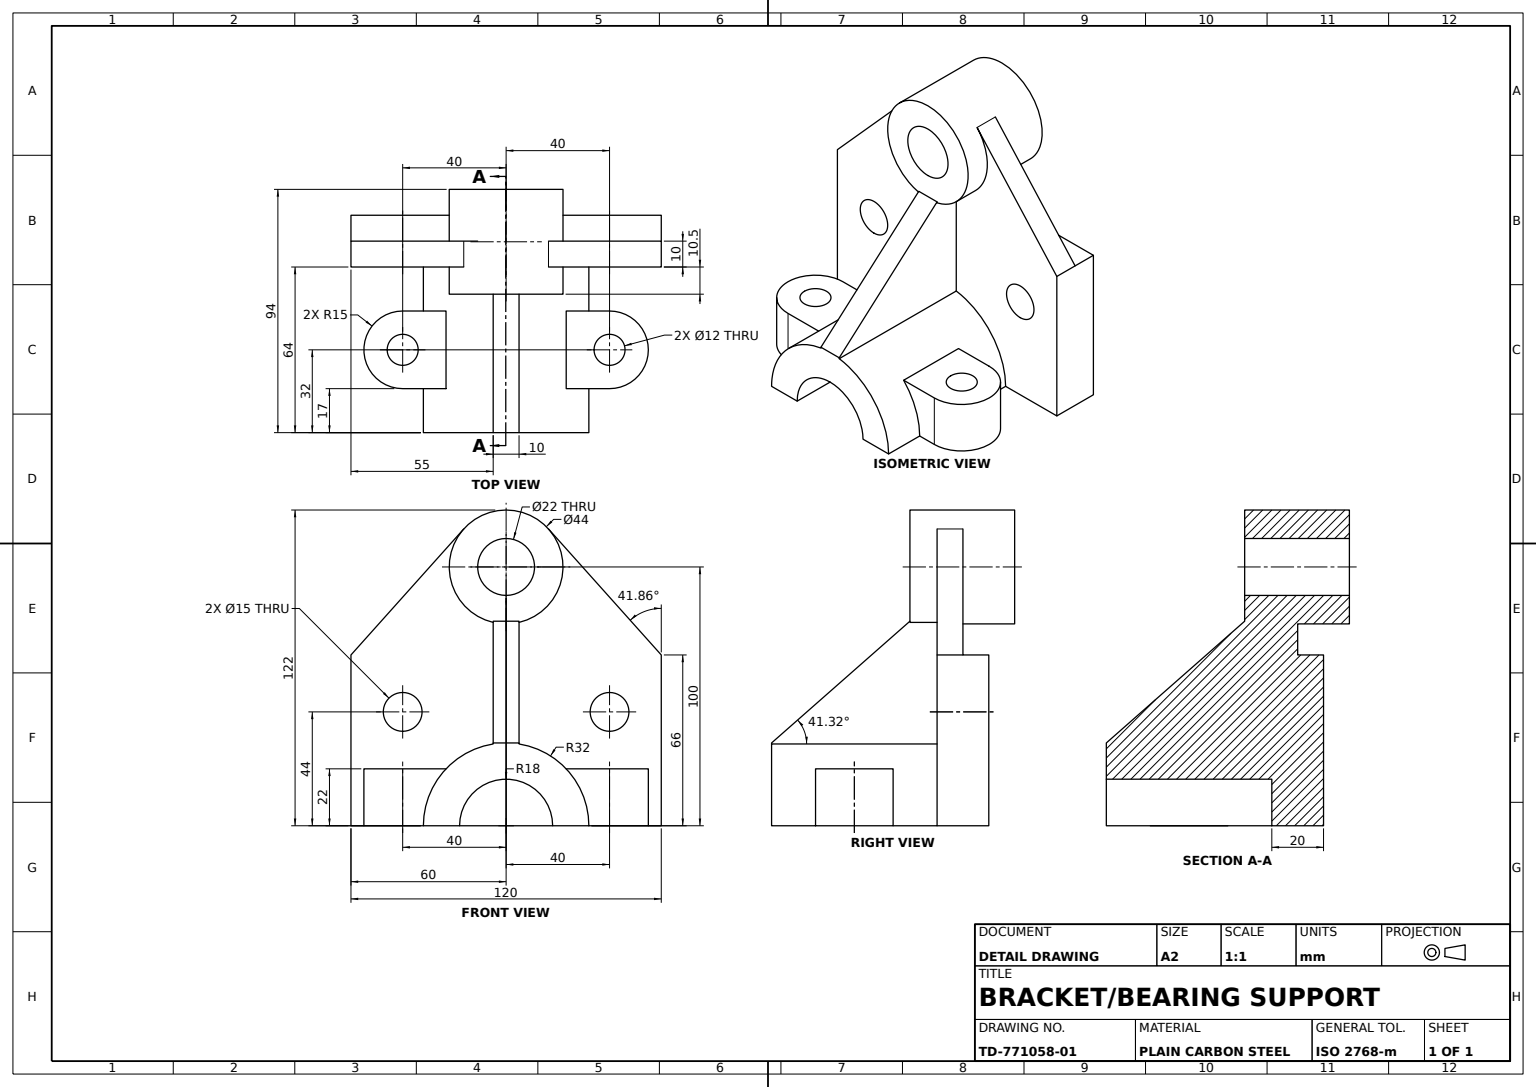
ISO-10303-21;
HEADER;
FILE_DESCRIPTION((''),'2;1');
FILE_NAME('','',(''),(''),'','','');
FILE_SCHEMA(('AUTOMOTIVE_DESIGN'));
ENDSEC;
DATA;
#1=APPLICATION_CONTEXT('');
#2=PRODUCT_CONTEXT('',#1,'mechanical');
#3=PRODUCT('','','',(#2));
#4=PRODUCT_DEFINITION_FORMATION('','',#3);
#5=PRODUCT_DEFINITION_CONTEXT('',#1,'design');
#6=PRODUCT_DEFINITION('','',#4,#5);
#7=PRODUCT_DEFINITION_SHAPE('','',#6);
#8=(LENGTH_UNIT()NAMED_UNIT(*)SI_UNIT(.MILLI.,.METRE.));
#9=(NAMED_UNIT(*)PLANE_ANGLE_UNIT()SI_UNIT($,.RADIAN.));
#10=(NAMED_UNIT(*)SI_UNIT($,.STERADIAN.)SOLID_ANGLE_UNIT());
#11=UNCERTAINTY_MEASURE_WITH_UNIT(LENGTH_MEASURE(1.E-05),#8,'distance_accuracy_value','');
#12=(GEOMETRIC_REPRESENTATION_CONTEXT(3)GLOBAL_UNCERTAINTY_ASSIGNED_CONTEXT((#11))GLOBAL_UNIT_ASSIGNED_CONTEXT((#8,#9,#10))REPRESENTATION_CONTEXT('',''));
#13=CARTESIAN_POINT('',(-10.,3.5,100.));
#14=VERTEX_POINT('',#13);
#15=CARTESIAN_POINT('',(-10.,18.5,100.));
#16=VERTEX_POINT('',#15);
#17=CARTESIAN_POINT('',(-10.,11.,100.));
#18=DIRECTION('',(1.,0.,0.));
#19=DIRECTION('',(0.,1.,0.));
#20=AXIS2_PLACEMENT_3D('',#17,#18,#19);
#21=CIRCLE('',#20,7.5);
#22=EDGE_CURVE('',#14,#16,#21,.T.);
#23=ORIENTED_EDGE('',*,*,#22,.F.);
#24=CARTESIAN_POINT('',(10.,3.5,100.));
#25=VERTEX_POINT('',#24);
#26=CARTESIAN_POINT('',(-20.,3.5,100.));
#27=VECTOR('',#18,1000.);
#28=LINE('',#26,#27);
#29=EDGE_CURVE('',#14,#25,#28,.T.);
#30=ORIENTED_EDGE('',*,*,#29,.T.);
#31=CARTESIAN_POINT('',(10.,18.5,100.));
#32=VERTEX_POINT('',#31);
#33=CARTESIAN_POINT('',(10.,11.,100.));
#34=AXIS2_PLACEMENT_3D('',#33,#18,#19);
#35=CIRCLE('',#34,7.5);
#36=EDGE_CURVE('',#25,#32,#35,.T.);
#37=ORIENTED_EDGE('',*,*,#36,.T.);
#38=CARTESIAN_POINT('',(-20.,18.5,100.));
#39=LINE('',#38,#27);
#40=EDGE_CURVE('',#16,#32,#39,.T.);
#41=ORIENTED_EDGE('',*,*,#40,.F.);
#42=EDGE_LOOP('',(#23,#30,#37,#41));
#43=FACE_OUTER_BOUND('',#42,.T.);
#44=CARTESIAN_POINT('',(-20.,11.,100.));
#45=AXIS2_PLACEMENT_3D('',#44,#18,#19);
#46=CYLINDRICAL_SURFACE('',#45,7.5);
#47=ADVANCED_FACE('',(#43),#46,.F.);
#48=CARTESIAN_POINT('',(74.,-1.393039,65.));
#49=VERTEX_POINT('',#48);
#50=CARTESIAN_POINT('',(74.,-33.,92.));
#51=VERTEX_POINT('',#50);
#52=CARTESIAN_POINT('',(74.,-33.,60.));
#53=AXIS2_PLACEMENT_3D('',#52,#18,#19);
#54=CIRCLE('',#53,32.);
#55=EDGE_CURVE('',#49,#51,#54,.T.);
#56=ORIENTED_EDGE('',*,*,#55,.F.);
#57=CARTESIAN_POINT('',(10.,-1.393039,65.));
#58=VERTEX_POINT('',#57);
#59=DIRECTION('',(-1.,0.,0.));
#60=VECTOR('',#59,1000.);
#61=LINE('',#48,#60);
#62=EDGE_CURVE('',#49,#58,#61,.T.);
#63=ORIENTED_EDGE('',*,*,#62,.T.);
#64=CARTESIAN_POINT('',(10.,-33.,92.));
#65=VERTEX_POINT('',#64);
#66=CARTESIAN_POINT('',(10.,-33.,60.));
#67=AXIS2_PLACEMENT_3D('',#66,#18,#19);
#68=CIRCLE('',#67,32.);
#69=EDGE_CURVE('',#58,#65,#68,.T.);
#70=ORIENTED_EDGE('',*,*,#69,.T.);
#71=CARTESIAN_POINT('',(27.,-33.,92.));
#72=VERTEX_POINT('',#71);
#73=LINE('',#50,#60);
#74=EDGE_CURVE('',#72,#65,#73,.T.);
#75=ORIENTED_EDGE('',*,*,#74,.F.);
#76=CARTESIAN_POINT('',(27.,-11.,83.2379));
#77=VERTEX_POINT('',#76);
#78=CARTESIAN_POINT('',(27.,-33.,60.));
#79=DIRECTION('',(0.,0.,1.));
#80=AXIS2_PLACEMENT_3D('',#78,#59,#79);
#81=CIRCLE('',#80,32.);
#82=EDGE_CURVE('',#72,#77,#81,.T.);
#83=ORIENTED_EDGE('',*,*,#82,.T.);
#84=CARTESIAN_POINT('',(57.,-11.,83.2379));
#85=VERTEX_POINT('',#84);
#86=CARTESIAN_POINT('',(74.,-11.,83.2379));
#87=LINE('',#86,#60);
#88=EDGE_CURVE('',#85,#77,#87,.T.);
#89=ORIENTED_EDGE('',*,*,#88,.F.);
#90=CARTESIAN_POINT('',(57.,-33.,92.));
#91=VERTEX_POINT('',#90);
#92=CARTESIAN_POINT('',(57.,-33.,60.));
#93=DIRECTION('',(0.,0.,-1.));
#94=AXIS2_PLACEMENT_3D('',#92,#18,#93);
#95=CIRCLE('',#94,32.);
#96=EDGE_CURVE('',#85,#91,#95,.T.);
#97=ORIENTED_EDGE('',*,*,#96,.T.);
#98=EDGE_CURVE('',#51,#91,#73,.T.);
#99=ORIENTED_EDGE('',*,*,#98,.F.);
#100=EDGE_LOOP('',(#56,#63,#70,#75,#83,#89,#97,#99));
#101=FACE_OUTER_BOUND('',#100,.T.);
#102=DIRECTION('',(0.,-1.,0.));
#103=AXIS2_PLACEMENT_3D('',#52,#59,#102);
#104=CYLINDRICAL_SURFACE('',#103,32.);
#105=ADVANCED_FACE('',(#101),#104,.T.);
#106=CARTESIAN_POINT('',(57.,-33.,28.));
#107=VERTEX_POINT('',#106);
#108=CARTESIAN_POINT('',(57.,-11.,36.7621));
#109=VERTEX_POINT('',#108);
#110=EDGE_CURVE('',#107,#109,#95,.T.);
#111=ORIENTED_EDGE('',*,*,#110,.F.);
#112=CARTESIAN_POINT('',(57.,-33.,20.));
#113=VERTEX_POINT('',#112);
#114=CARTESIAN_POINT('',(57.,-33.,38.));
#115=VECTOR('',#79,1000.);
#116=LINE('',#114,#115);
#117=EDGE_CURVE('',#113,#107,#116,.T.);
#118=ORIENTED_EDGE('',*,*,#117,.F.);
#119=CARTESIAN_POINT('',(57.,-11.,20.));
#120=VERTEX_POINT('',#119);
#121=VECTOR('',#102,1000.);
#122=LINE('',#119,#121);
#123=EDGE_CURVE('',#120,#113,#122,.T.);
#124=ORIENTED_EDGE('',*,*,#123,.F.);
#125=CARTESIAN_POINT('',(57.,-11.,35.));
#126=LINE('',#125,#115);
#127=EDGE_CURVE('',#120,#109,#126,.T.);
#128=ORIENTED_EDGE('',*,*,#127,.T.);
#129=EDGE_LOOP('',(#111,#118,#124,#128));
#130=FACE_OUTER_BOUND('',#129,.T.);
#131=CARTESIAN_POINT('',(57.,-11.,38.));
#132=AXIS2_PLACEMENT_3D('',#131,#18,#93);
#133=PLANE('',#132);
#134=ADVANCED_FACE('',(#130),#133,.T.);
#135=CARTESIAN_POINT('',(42.,-33.,5.));
#136=VERTEX_POINT('',#135);
#137=CARTESIAN_POINT('',(42.,-33.,20.));
#138=AXIS2_PLACEMENT_3D('',#137,#102,#93);
#139=CIRCLE('',#138,15.);
#140=EDGE_CURVE('',#136,#113,#139,.T.);
#141=ORIENTED_EDGE('',*,*,#140,.T.);
#142=ORIENTED_EDGE('',*,*,#117,.T.);
#143=CARTESIAN_POINT('',(74.,-33.,28.));
#144=VERTEX_POINT('',#143);
#145=LINE('',#143,#60);
#146=EDGE_CURVE('',#144,#107,#145,.T.);
#147=ORIENTED_EDGE('',*,*,#146,.F.);
#148=CARTESIAN_POINT('',(74.,-33.,42.));
#149=VERTEX_POINT('',#148);
#150=VECTOR('',#93,1000.);
#151=LINE('',#148,#150);
#152=EDGE_CURVE('',#149,#144,#151,.T.);
#153=ORIENTED_EDGE('',*,*,#152,.F.);
#154=CARTESIAN_POINT('',(10.,-33.,42.));
#155=VERTEX_POINT('',#154);
#156=LINE('',#148,#60);
#157=EDGE_CURVE('',#149,#155,#156,.T.);
#158=ORIENTED_EDGE('',*,*,#157,.T.);
#159=CARTESIAN_POINT('',(10.,-33.,78.));
#160=VERTEX_POINT('',#159);
#161=CARTESIAN_POINT('',(10.,-33.,120.));
#162=LINE('',#161,#150);
#163=EDGE_CURVE('',#160,#155,#162,.T.);
#164=ORIENTED_EDGE('',*,*,#163,.F.);
#165=CARTESIAN_POINT('',(74.,-33.,78.));
#166=VERTEX_POINT('',#165);
#167=LINE('',#165,#60);
#168=EDGE_CURVE('',#166,#160,#167,.T.);
#169=ORIENTED_EDGE('',*,*,#168,.F.);
#170=LINE('',#50,#150);
#171=EDGE_CURVE('',#51,#166,#170,.T.);
#172=ORIENTED_EDGE('',*,*,#171,.F.);
#173=ORIENTED_EDGE('',*,*,#98,.T.);
#174=CARTESIAN_POINT('',(57.,-33.,100.));
#175=VERTEX_POINT('',#174);
#176=CARTESIAN_POINT('',(57.,-33.,85.));
#177=LINE('',#176,#115);
#178=EDGE_CURVE('',#91,#175,#177,.T.);
#179=ORIENTED_EDGE('',*,*,#178,.T.);
#180=CARTESIAN_POINT('',(27.,-33.,100.));
#181=VERTEX_POINT('',#180);
#182=CARTESIAN_POINT('',(42.,-33.,100.));
#183=AXIS2_PLACEMENT_3D('',#182,#102,#93);
#184=CIRCLE('',#183,15.);
#185=EDGE_CURVE('',#175,#181,#184,.T.);
#186=ORIENTED_EDGE('',*,*,#185,.T.);
#187=LINE('',#180,#150);
#188=EDGE_CURVE('',#181,#72,#187,.T.);
#189=ORIENTED_EDGE('',*,*,#188,.T.);
#190=ORIENTED_EDGE('',*,*,#74,.T.);
#191=VERTEX_POINT('',#161);
#192=EDGE_CURVE('',#191,#65,#162,.T.);
#193=ORIENTED_EDGE('',*,*,#192,.F.);
#194=CARTESIAN_POINT('',(-10.,-33.,120.));
#195=VERTEX_POINT('',#194);
#196=LINE('',#194,#27);
#197=EDGE_CURVE('',#195,#191,#196,.T.);
#198=ORIENTED_EDGE('',*,*,#197,.F.);
#199=CARTESIAN_POINT('',(-10.,-33.,0.));
#200=VERTEX_POINT('',#199);
#201=LINE('',#194,#150);
#202=EDGE_CURVE('',#195,#200,#201,.T.);
#203=ORIENTED_EDGE('',*,*,#202,.T.);
#204=CARTESIAN_POINT('',(10.,-33.,0.));
#205=VERTEX_POINT('',#204);
#206=LINE('',#199,#27);
#207=EDGE_CURVE('',#200,#205,#206,.T.);
#208=ORIENTED_EDGE('',*,*,#207,.T.);
#209=CARTESIAN_POINT('',(10.,-33.,28.));
#210=VERTEX_POINT('',#209);
#211=EDGE_CURVE('',#210,#205,#162,.T.);
#212=ORIENTED_EDGE('',*,*,#211,.F.);
#213=CARTESIAN_POINT('',(27.,-33.,28.));
#214=VERTEX_POINT('',#213);
#215=EDGE_CURVE('',#214,#210,#145,.T.);
#216=ORIENTED_EDGE('',*,*,#215,.F.);
#217=CARTESIAN_POINT('',(27.,-33.,20.));
#218=VERTEX_POINT('',#217);
#219=LINE('',#217,#150);
#220=EDGE_CURVE('',#214,#218,#219,.T.);
#221=ORIENTED_EDGE('',*,*,#220,.T.);
#222=EDGE_CURVE('',#218,#136,#139,.T.);
#223=ORIENTED_EDGE('',*,*,#222,.T.);
#224=EDGE_LOOP('',(#141,#142,#147,#153,#158,#164,#169,#172,#173,#179,#186,#189,#190,#193,#198,#203,#208,#212,#216,#221,#223));
#225=FACE_OUTER_BOUND('',#224,.T.);
#226=CARTESIAN_POINT('',(42.,-33.,26.));
#227=VERTEX_POINT('',#226);
#228=CARTESIAN_POINT('',(42.,-33.,14.));
#229=VERTEX_POINT('',#228);
#230=CIRCLE('',#138,6.);
#231=EDGE_CURVE('',#227,#229,#230,.T.);
#232=ORIENTED_EDGE('',*,*,#231,.F.);
#233=EDGE_CURVE('',#229,#227,#230,.T.);
#234=ORIENTED_EDGE('',*,*,#233,.F.);
#235=EDGE_LOOP('',(#232,#234));
#236=FACE_BOUND('',#235,.T.);
#237=CARTESIAN_POINT('',(42.,-33.,94.));
#238=VERTEX_POINT('',#237);
#239=CARTESIAN_POINT('',(42.,-33.,106.));
#240=VERTEX_POINT('',#239);
#241=CIRCLE('',#183,6.);
#242=EDGE_CURVE('',#238,#240,#241,.T.);
#243=ORIENTED_EDGE('',*,*,#242,.F.);
#244=EDGE_CURVE('',#240,#238,#241,.T.);
#245=ORIENTED_EDGE('',*,*,#244,.F.);
#246=EDGE_LOOP('',(#243,#245));
#247=FACE_BOUND('',#246,.T.);
#248=AXIS2_PLACEMENT_3D('',#194,#19,#79);
#249=PLANE('',#248);
#250=ADVANCED_FACE('',(#225,#236,#247),#249,.F.);
#251=CARTESIAN_POINT('',(10.,33.,120.));
#252=VERTEX_POINT('',#251);
#253=CARTESIAN_POINT('',(10.,81.680385,76.385551));
#254=VERTEX_POINT('',#253);
#255=CARTESIAN_POINT('',(10.,74.333671,82.967728));
#256=DIRECTION('',(0.,0.744797795,-0.667290226));
#257=VECTOR('',#256,1000.);
#258=LINE('',#255,#257);
#259=EDGE_CURVE('',#252,#254,#258,.T.);
#260=ORIENTED_EDGE('',*,*,#259,.T.);
#261=CARTESIAN_POINT('',(0.,81.680385,76.385551));
#262=VERTEX_POINT('',#261);
#263=LINE('',#261,#27);
#264=EDGE_CURVE('',#262,#254,#263,.T.);
#265=ORIENTED_EDGE('',*,*,#264,.F.);
#266=CARTESIAN_POINT('',(0.,33.,120.));
#267=VERTEX_POINT('',#266);
#268=CARTESIAN_POINT('',(0.,74.333671,82.967728));
#269=LINE('',#268,#257);
#270=EDGE_CURVE('',#267,#262,#269,.T.);
#271=ORIENTED_EDGE('',*,*,#270,.F.);
#272=CARTESIAN_POINT('',(-10.,33.,120.));
#273=LINE('',#272,#60);
#274=EDGE_CURVE('',#252,#267,#273,.T.);
#275=ORIENTED_EDGE('',*,*,#274,.F.);
#276=EDGE_LOOP('',(#260,#265,#271,#275));
#277=FACE_OUTER_BOUND('',#276,.T.);
#278=DIRECTION('',(0.,-0.667290226,-0.744797795));
#279=AXIS2_PLACEMENT_3D('',#268,#278,#256);
#280=PLANE('',#279);
#281=ADVANCED_FACE('',(#277),#280,.F.);
#282=CARTESIAN_POINT('',(-10.,3.5,20.));
#283=VERTEX_POINT('',#282);
#284=CARTESIAN_POINT('',(-10.,18.5,20.));
#285=VERTEX_POINT('',#284);
#286=CARTESIAN_POINT('',(-10.,11.,20.));
#287=AXIS2_PLACEMENT_3D('',#286,#18,#19);
#288=CIRCLE('',#287,7.5);
#289=EDGE_CURVE('',#283,#285,#288,.T.);
#290=ORIENTED_EDGE('',*,*,#289,.F.);
#291=CARTESIAN_POINT('',(10.,3.5,20.));
#292=VERTEX_POINT('',#291);
#293=CARTESIAN_POINT('',(-20.,3.5,20.));
#294=LINE('',#293,#27);
#295=EDGE_CURVE('',#283,#292,#294,.T.);
#296=ORIENTED_EDGE('',*,*,#295,.T.);
#297=CARTESIAN_POINT('',(10.,18.5,20.));
#298=VERTEX_POINT('',#297);
#299=CARTESIAN_POINT('',(10.,11.,20.));
#300=AXIS2_PLACEMENT_3D('',#299,#18,#19);
#301=CIRCLE('',#300,7.5);
#302=EDGE_CURVE('',#292,#298,#301,.T.);
#303=ORIENTED_EDGE('',*,*,#302,.T.);
#304=CARTESIAN_POINT('',(-20.,18.5,20.));
#305=LINE('',#304,#27);
#306=EDGE_CURVE('',#285,#298,#305,.T.);
#307=ORIENTED_EDGE('',*,*,#306,.F.);
#308=EDGE_LOOP('',(#290,#296,#303,#307));
#309=FACE_OUTER_BOUND('',#308,.T.);
#310=CARTESIAN_POINT('',(-20.,11.,20.));
#311=AXIS2_PLACEMENT_3D('',#310,#18,#19);
#312=CYLINDRICAL_SURFACE('',#311,7.5);
#313=ADVANCED_FACE('',(#309),#312,.F.);
#314=CARTESIAN_POINT('',(42.,-11.,94.));
#315=VERTEX_POINT('',#314);
#316=CARTESIAN_POINT('',(42.,-11.,106.));
#317=VERTEX_POINT('',#316);
#318=CARTESIAN_POINT('',(42.,-11.,100.));
#319=AXIS2_PLACEMENT_3D('',#318,#102,#93);
#320=CIRCLE('',#319,6.);
#321=EDGE_CURVE('',#315,#317,#320,.T.);
#322=ORIENTED_EDGE('',*,*,#321,.T.);
#323=EDGE_CURVE('',#317,#315,#320,.T.);
#324=ORIENTED_EDGE('',*,*,#323,.T.);
#325=EDGE_LOOP('',(#322,#324));
#326=FACE_BOUND('',#325,.T.);
#327=CARTESIAN_POINT('',(27.,-11.,100.));
#328=VERTEX_POINT('',#327);
#329=LINE('',#327,#150);
#330=EDGE_CURVE('',#328,#77,#329,.T.);
#331=ORIENTED_EDGE('',*,*,#330,.F.);
#332=CARTESIAN_POINT('',(57.,-11.,100.));
#333=VERTEX_POINT('',#332);
#334=CIRCLE('',#319,15.);
#335=EDGE_CURVE('',#333,#328,#334,.T.);
#336=ORIENTED_EDGE('',*,*,#335,.F.);
#337=CARTESIAN_POINT('',(57.,-11.,83.));
#338=LINE('',#337,#115);
#339=EDGE_CURVE('',#85,#333,#338,.T.);
#340=ORIENTED_EDGE('',*,*,#339,.F.);
#341=ORIENTED_EDGE('',*,*,#88,.T.);
#342=EDGE_LOOP('',(#331,#336,#340,#341));
#343=FACE_OUTER_BOUND('',#342,.T.);
#344=PLANE('',#319);
#345=ADVANCED_FACE('',(#326,#343),#344,.F.);
#346=CARTESIAN_POINT('',(-20.,45.,60.));
#347=VERTEX_POINT('',#346);
#348=CARTESIAN_POINT('',(0.,45.,60.));
#349=VERTEX_POINT('',#348);
#350=LINE('',#348,#27);
#351=EDGE_CURVE('',#347,#349,#350,.T.);
#352=ORIENTED_EDGE('',*,*,#351,.T.);
#353=CARTESIAN_POINT('',(0.,67.,60.));
#354=AXIS2_PLACEMENT_3D('',#353,#59,#19);
#355=CIRCLE('',#354,22.);
#356=EDGE_CURVE('',#349,#262,#355,.T.);
#357=ORIENTED_EDGE('',*,*,#356,.T.);
#358=ORIENTED_EDGE('',*,*,#264,.T.);
#359=CARTESIAN_POINT('',(10.,45.575715,65.));
#360=VERTEX_POINT('',#359);
#361=CARTESIAN_POINT('',(10.,67.,60.));
#362=AXIS2_PLACEMENT_3D('',#361,#18,#19);
#363=CIRCLE('',#362,22.);
#364=EDGE_CURVE('',#254,#360,#363,.T.);
#365=ORIENTED_EDGE('',*,*,#364,.T.);
#366=CARTESIAN_POINT('',(20.5,45.575715,65.));
#367=VERTEX_POINT('',#366);
#368=CARTESIAN_POINT('',(0.,45.575715,65.));
#369=LINE('',#368,#60);
#370=EDGE_CURVE('',#367,#360,#369,.T.);
#371=ORIENTED_EDGE('',*,*,#370,.F.);
#372=CARTESIAN_POINT('',(20.5,89.,60.));
#373=VERTEX_POINT('',#372);
#374=CARTESIAN_POINT('',(20.5,67.,60.));
#375=AXIS2_PLACEMENT_3D('',#374,#18,#19);
#376=CIRCLE('',#375,22.);
#377=EDGE_CURVE('',#373,#367,#376,.T.);
#378=ORIENTED_EDGE('',*,*,#377,.F.);
#379=CARTESIAN_POINT('',(-20.,89.,60.));
#380=VERTEX_POINT('',#379);
#381=CARTESIAN_POINT('',(0.,89.,60.));
#382=LINE('',#381,#27);
#383=EDGE_CURVE('',#380,#373,#382,.T.);
#384=ORIENTED_EDGE('',*,*,#383,.F.);
#385=CARTESIAN_POINT('',(-20.,67.,60.));
#386=AXIS2_PLACEMENT_3D('',#385,#59,#102);
#387=CIRCLE('',#386,22.);
#388=EDGE_CURVE('',#347,#380,#387,.T.);
#389=ORIENTED_EDGE('',*,*,#388,.F.);
#390=EDGE_LOOP('',(#352,#357,#358,#365,#371,#378,#384,#389));
#391=FACE_OUTER_BOUND('',#390,.T.);
#392=AXIS2_PLACEMENT_3D('',#353,#18,#19);
#393=CYLINDRICAL_SURFACE('',#392,22.);
#394=ADVANCED_FACE('',(#391),#393,.T.);
#395=ORIENTED_EDGE('',*,*,#123,.T.);
#396=ORIENTED_EDGE('',*,*,#140,.F.);
#397=CARTESIAN_POINT('',(42.,-11.,5.));
#398=VERTEX_POINT('',#397);
#399=LINE('',#397,#121);
#400=EDGE_CURVE('',#398,#136,#399,.T.);
#401=ORIENTED_EDGE('',*,*,#400,.F.);
#402=CARTESIAN_POINT('',(42.,-11.,20.));
#403=AXIS2_PLACEMENT_3D('',#402,#102,#93);
#404=CIRCLE('',#403,15.);
#405=EDGE_CURVE('',#398,#120,#404,.T.);
#406=ORIENTED_EDGE('',*,*,#405,.T.);
#407=EDGE_LOOP('',(#395,#396,#401,#406));
#408=FACE_OUTER_BOUND('',#407,.T.);
#409=CYLINDRICAL_SURFACE('',#403,15.);
#410=ADVANCED_FACE('',(#408),#409,.T.);
#411=ORIENTED_EDGE('',*,*,#157,.F.);
#412=AXIS2_PLACEMENT_3D('',#52,#59,#19);
#413=CIRCLE('',#412,18.);
#414=EDGE_CURVE('',#166,#149,#413,.T.);
#415=ORIENTED_EDGE('',*,*,#414,.F.);
#416=ORIENTED_EDGE('',*,*,#168,.T.);
#417=AXIS2_PLACEMENT_3D('',#66,#59,#19);
#418=CIRCLE('',#417,18.);
#419=EDGE_CURVE('',#160,#155,#418,.T.);
#420=ORIENTED_EDGE('',*,*,#419,.T.);
#421=EDGE_LOOP('',(#411,#415,#416,#420));
#422=FACE_OUTER_BOUND('',#421,.T.);
#423=CYLINDRICAL_SURFACE('',#103,18.);
#424=ADVANCED_FACE('',(#422),#423,.F.);
#425=CARTESIAN_POINT('',(10.,45.575715,55.));
#426=VERTEX_POINT('',#425);
#427=CARTESIAN_POINT('',(10.,81.680385,43.614449));
#428=VERTEX_POINT('',#427);
#429=EDGE_CURVE('',#426,#428,#363,.T.);
#430=ORIENTED_EDGE('',*,*,#429,.F.);
#431=CARTESIAN_POINT('',(10.,-1.393039,55.));
#432=VERTEX_POINT('',#431);
#433=CARTESIAN_POINT('',(10.,-5.,55.));
#434=LINE('',#433,#121);
#435=EDGE_CURVE('',#426,#432,#434,.T.);
#436=ORIENTED_EDGE('',*,*,#435,.T.);
#437=EDGE_CURVE('',#210,#432,#68,.T.);
#438=ORIENTED_EDGE('',*,*,#437,.F.);
#439=ORIENTED_EDGE('',*,*,#211,.T.);
#440=CARTESIAN_POINT('',(10.,33.,0.));
#441=VERTEX_POINT('',#440);
#442=VECTOR('',#19,1000.);
#443=LINE('',#440,#442);
#444=EDGE_CURVE('',#205,#441,#443,.T.);
#445=ORIENTED_EDGE('',*,*,#444,.T.);
#446=CARTESIAN_POINT('',(10.,14.694116,-16.400878));
#447=DIRECTION('',(0.,0.744797795,0.667290226));
#448=VECTOR('',#447,1000.);
#449=LINE('',#446,#448);
#450=EDGE_CURVE('',#441,#428,#449,.T.);
#451=ORIENTED_EDGE('',*,*,#450,.T.);
#452=EDGE_LOOP('',(#430,#436,#438,#439,#445,#451));
#453=FACE_OUTER_BOUND('',#452,.T.);
#454=EDGE_CURVE('',#298,#292,#301,.T.);
#455=ORIENTED_EDGE('',*,*,#454,.F.);
#456=ORIENTED_EDGE('',*,*,#302,.F.);
#457=EDGE_LOOP('',(#455,#456));
#458=FACE_BOUND('',#457,.T.);
#459=AXIS2_PLACEMENT_3D('',#251,#59,#102);
#460=PLANE('',#459);
#461=ADVANCED_FACE('',(#453,#458),#460,.F.);
#462=LINE('',#314,#121);
#463=EDGE_CURVE('',#315,#238,#462,.T.);
#464=ORIENTED_EDGE('',*,*,#463,.F.);
#465=ORIENTED_EDGE('',*,*,#323,.F.);
#466=LINE('',#316,#121);
#467=EDGE_CURVE('',#317,#240,#466,.T.);
#468=ORIENTED_EDGE('',*,*,#467,.T.);
#469=ORIENTED_EDGE('',*,*,#244,.T.);
#470=EDGE_LOOP('',(#464,#465,#468,#469));
#471=FACE_OUTER_BOUND('',#470,.T.);
#472=CYLINDRICAL_SURFACE('',#319,6.);
#473=ADVANCED_FACE('',(#471),#472,.F.);
#474=ORIENTED_EDGE('',*,*,#82,.F.);
#475=ORIENTED_EDGE('',*,*,#188,.F.);
#476=LINE('',#327,#121);
#477=EDGE_CURVE('',#328,#181,#476,.T.);
#478=ORIENTED_EDGE('',*,*,#477,.F.);
#479=ORIENTED_EDGE('',*,*,#330,.T.);
#480=EDGE_LOOP('',(#474,#475,#478,#479));
#481=FACE_OUTER_BOUND('',#480,.T.);
#482=AXIS2_PLACEMENT_3D('',#327,#59,#79);
#483=PLANE('',#482);
#484=ADVANCED_FACE('',(#481),#483,.T.);
#485=CARTESIAN_POINT('',(20.5,46.039175,55.));
#486=VERTEX_POINT('',#485);
#487=CARTESIAN_POINT('',(20.5,46.039175,65.));
#488=VERTEX_POINT('',#487);
#489=LINE('',#487,#115);
#490=EDGE_CURVE('',#486,#488,#489,.T.);
#491=ORIENTED_EDGE('',*,*,#490,.T.);
#492=CARTESIAN_POINT('',(74.,-1.,65.));
#493=VERTEX_POINT('',#492);
#494=CARTESIAN_POINT('',(20.,46.478793,65.));
#495=DIRECTION('',(-0.750997662,0.660304863,0.));
#496=VECTOR('',#495,1000.);
#497=LINE('',#494,#496);
#498=EDGE_CURVE('',#493,#488,#497,.T.);
#499=ORIENTED_EDGE('',*,*,#498,.F.);
#500=CARTESIAN_POINT('',(74.,-1.,55.));
#501=VERTEX_POINT('',#500);
#502=LINE('',#492,#150);
#503=EDGE_CURVE('',#493,#501,#502,.T.);
#504=ORIENTED_EDGE('',*,*,#503,.T.);
#505=CARTESIAN_POINT('',(20.,46.478793,55.));
#506=LINE('',#505,#496);
#507=EDGE_CURVE('',#501,#486,#506,.T.);
#508=ORIENTED_EDGE('',*,*,#507,.T.);
#509=EDGE_LOOP('',(#491,#499,#504,#508));
#510=FACE_OUTER_BOUND('',#509,.T.);
#511=DIRECTION('',(-0.660304863,-0.750997662,0.));
#512=DIRECTION('',(0.750997662,-0.660304863,0.));
#513=AXIS2_PLACEMENT_3D('',#494,#511,#512);
#514=PLANE('',#513);
#515=ADVANCED_FACE('',(#510),#514,.F.);
#516=VERTEX_POINT('',#272);
#517=EDGE_CURVE('',#267,#516,#273,.T.);
#518=ORIENTED_EDGE('',*,*,#517,.F.);
#519=CARTESIAN_POINT('',(0.,33.,0.));
#520=VERTEX_POINT('',#519);
#521=LINE('',#519,#115);
#522=EDGE_CURVE('',#520,#267,#521,.T.);
#523=ORIENTED_EDGE('',*,*,#522,.F.);
#524=CARTESIAN_POINT('',(-10.,33.,0.));
#525=VERTEX_POINT('',#524);
#526=LINE('',#524,#60);
#527=EDGE_CURVE('',#520,#525,#526,.T.);
#528=ORIENTED_EDGE('',*,*,#527,.T.);
#529=LINE('',#272,#150);
#530=EDGE_CURVE('',#516,#525,#529,.T.);
#531=ORIENTED_EDGE('',*,*,#530,.F.);
#532=EDGE_LOOP('',(#518,#523,#528,#531));
#533=FACE_OUTER_BOUND('',#532,.T.);
#534=AXIS2_PLACEMENT_3D('',#272,#102,#18);
#535=PLANE('',#534);
#536=ADVANCED_FACE('',(#533),#535,.F.);
#537=CARTESIAN_POINT('',(27.,-11.,20.));
#538=VERTEX_POINT('',#537);
#539=LINE('',#537,#121);
#540=EDGE_CURVE('',#538,#218,#539,.T.);
#541=ORIENTED_EDGE('',*,*,#540,.T.);
#542=ORIENTED_EDGE('',*,*,#220,.F.);
#543=CARTESIAN_POINT('',(27.,-11.,36.7621));
#544=VERTEX_POINT('',#543);
#545=EDGE_CURVE('',#544,#214,#81,.T.);
#546=ORIENTED_EDGE('',*,*,#545,.F.);
#547=LINE('',#537,#150);
#548=EDGE_CURVE('',#544,#538,#547,.T.);
#549=ORIENTED_EDGE('',*,*,#548,.T.);
#550=EDGE_LOOP('',(#541,#542,#546,#549));
#551=FACE_OUTER_BOUND('',#550,.T.);
#552=AXIS2_PLACEMENT_3D('',#537,#59,#79);
#553=PLANE('',#552);
#554=ADVANCED_FACE('',(#551),#553,.T.);
#555=ORIENTED_EDGE('',*,*,#295,.F.);
#556=EDGE_CURVE('',#285,#283,#288,.T.);
#557=ORIENTED_EDGE('',*,*,#556,.F.);
#558=ORIENTED_EDGE('',*,*,#306,.T.);
#559=ORIENTED_EDGE('',*,*,#454,.T.);
#560=EDGE_LOOP('',(#555,#557,#558,#559));
#561=FACE_OUTER_BOUND('',#560,.T.);
#562=ADVANCED_FACE('',(#561),#312,.F.);
#563=ORIENTED_EDGE('',*,*,#339,.T.);
#564=LINE('',#332,#121);
#565=EDGE_CURVE('',#333,#175,#564,.T.);
#566=ORIENTED_EDGE('',*,*,#565,.T.);
#567=ORIENTED_EDGE('',*,*,#178,.F.);
#568=ORIENTED_EDGE('',*,*,#96,.F.);
#569=EDGE_LOOP('',(#563,#566,#567,#568));
#570=FACE_OUTER_BOUND('',#569,.T.);
#571=CARTESIAN_POINT('',(57.,-11.,85.));
#572=AXIS2_PLACEMENT_3D('',#571,#18,#93);
#573=PLANE('',#572);
#574=ADVANCED_FACE('',(#570),#573,.T.);
#575=CARTESIAN_POINT('',(0.,81.680385,43.614449));
#576=VERTEX_POINT('',#575);
#577=CARTESIAN_POINT('',(0.,14.694116,-16.400878));
#578=LINE('',#577,#448);
#579=EDGE_CURVE('',#520,#576,#578,.T.);
#580=ORIENTED_EDGE('',*,*,#579,.T.);
#581=LINE('',#575,#27);
#582=EDGE_CURVE('',#576,#428,#581,.T.);
#583=ORIENTED_EDGE('',*,*,#582,.T.);
#584=ORIENTED_EDGE('',*,*,#450,.F.);
#585=EDGE_CURVE('',#441,#520,#526,.T.);
#586=ORIENTED_EDGE('',*,*,#585,.T.);
#587=EDGE_LOOP('',(#580,#583,#584,#586));
#588=FACE_OUTER_BOUND('',#587,.T.);
#589=DIRECTION('',(0.,0.667290226,-0.744797795));
#590=AXIS2_PLACEMENT_3D('',#577,#589,#447);
#591=PLANE('',#590);
#592=ADVANCED_FACE('',(#588),#591,.T.);
#593=CARTESIAN_POINT('',(42.,-11.,14.));
#594=VERTEX_POINT('',#593);
#595=LINE('',#593,#121);
#596=EDGE_CURVE('',#594,#229,#595,.T.);
#597=ORIENTED_EDGE('',*,*,#596,.F.);
#598=CARTESIAN_POINT('',(42.,-11.,26.));
#599=VERTEX_POINT('',#598);
#600=CIRCLE('',#403,6.);
#601=EDGE_CURVE('',#599,#594,#600,.T.);
#602=ORIENTED_EDGE('',*,*,#601,.F.);
#603=LINE('',#598,#121);
#604=EDGE_CURVE('',#599,#227,#603,.T.);
#605=ORIENTED_EDGE('',*,*,#604,.T.);
#606=ORIENTED_EDGE('',*,*,#231,.T.);
#607=EDGE_LOOP('',(#597,#602,#605,#606));
#608=FACE_OUTER_BOUND('',#607,.T.);
#609=CYLINDRICAL_SURFACE('',#403,6.);
#610=ADVANCED_FACE('',(#608),#609,.F.);
#611=ORIENTED_EDGE('',*,*,#498,.T.);
#612=CARTESIAN_POINT('',(20.5,0.,65.));
#613=LINE('',#612,#442);
#614=EDGE_CURVE('',#367,#488,#613,.T.);
#615=ORIENTED_EDGE('',*,*,#614,.F.);
#616=ORIENTED_EDGE('',*,*,#370,.T.);
#617=CARTESIAN_POINT('',(10.,-5.,65.));
#618=LINE('',#617,#121);
#619=EDGE_CURVE('',#360,#58,#618,.T.);
#620=ORIENTED_EDGE('',*,*,#619,.T.);
#621=ORIENTED_EDGE('',*,*,#62,.F.);
#622=CARTESIAN_POINT('',(74.,-5.,65.));
#623=LINE('',#622,#442);
#624=EDGE_CURVE('',#49,#493,#623,.T.);
#625=ORIENTED_EDGE('',*,*,#624,.T.);
#626=EDGE_LOOP('',(#611,#615,#616,#620,#621,#625));
#627=FACE_OUTER_BOUND('',#626,.T.);
#628=CARTESIAN_POINT('',(0.,0.,65.));
#629=AXIS2_PLACEMENT_3D('',#628,#79,#18);
#630=PLANE('',#629);
#631=ADVANCED_FACE('',(#627),#630,.T.);
#632=ORIENTED_EDGE('',*,*,#429,.T.);
#633=ORIENTED_EDGE('',*,*,#582,.F.);
#634=EDGE_CURVE('',#576,#349,#355,.T.);
#635=ORIENTED_EDGE('',*,*,#634,.T.);
#636=ORIENTED_EDGE('',*,*,#351,.F.);
#637=EDGE_CURVE('',#380,#347,#387,.T.);
#638=ORIENTED_EDGE('',*,*,#637,.F.);
#639=ORIENTED_EDGE('',*,*,#383,.T.);
#640=CARTESIAN_POINT('',(20.5,45.575715,55.));
#641=VERTEX_POINT('',#640);
#642=EDGE_CURVE('',#641,#373,#376,.T.);
#643=ORIENTED_EDGE('',*,*,#642,.F.);
#644=CARTESIAN_POINT('',(0.,45.575715,55.));
#645=LINE('',#644,#60);
#646=EDGE_CURVE('',#641,#426,#645,.T.);
#647=ORIENTED_EDGE('',*,*,#646,.T.);
#648=EDGE_LOOP('',(#632,#633,#635,#636,#638,#639,#643,#647));
#649=FACE_OUTER_BOUND('',#648,.T.);
#650=ADVANCED_FACE('',(#649),#393,.T.);
#651=ORIENTED_EDGE('',*,*,#400,.T.);
#652=ORIENTED_EDGE('',*,*,#222,.F.);
#653=ORIENTED_EDGE('',*,*,#540,.F.);
#654=EDGE_CURVE('',#538,#398,#404,.T.);
#655=ORIENTED_EDGE('',*,*,#654,.T.);
#656=EDGE_LOOP('',(#651,#652,#653,#655));
#657=FACE_OUTER_BOUND('',#656,.T.);
#658=ADVANCED_FACE('',(#657),#409,.T.);
#659=ORIENTED_EDGE('',*,*,#163,.T.);
#660=ORIENTED_EDGE('',*,*,#419,.F.);
#661=EDGE_LOOP('',(#659,#660));
#662=FACE_OUTER_BOUND('',#661,.T.);
#663=ADVANCED_FACE('',(#662),#460,.F.);
#664=LINE('',#272,#121);
#665=EDGE_CURVE('',#516,#195,#664,.T.);
#666=ORIENTED_EDGE('',*,*,#665,.T.);
#667=ORIENTED_EDGE('',*,*,#197,.T.);
#668=LINE('',#251,#442);
#669=EDGE_CURVE('',#191,#252,#668,.T.);
#670=ORIENTED_EDGE('',*,*,#669,.T.);
#671=ORIENTED_EDGE('',*,*,#274,.T.);
#672=ORIENTED_EDGE('',*,*,#517,.T.);
#673=EDGE_LOOP('',(#666,#667,#670,#671,#672));
#674=FACE_OUTER_BOUND('',#673,.T.);
#675=CARTESIAN_POINT('',(0.,0.,120.));
#676=AXIS2_PLACEMENT_3D('',#675,#79,#18);
#677=PLANE('',#676);
#678=ADVANCED_FACE('',(#674),#677,.T.);
#679=CARTESIAN_POINT('',(-20.,56.,60.));
#680=VERTEX_POINT('',#679);
#681=CARTESIAN_POINT('',(-20.,78.,60.));
#682=VERTEX_POINT('',#681);
#683=CIRCLE('',#386,11.);
#684=EDGE_CURVE('',#680,#682,#683,.T.);
#685=ORIENTED_EDGE('',*,*,#684,.T.);
#686=CARTESIAN_POINT('',(20.5,78.,60.));
#687=VERTEX_POINT('',#686);
#688=CARTESIAN_POINT('',(0.,78.,60.));
#689=LINE('',#688,#27);
#690=EDGE_CURVE('',#682,#687,#689,.T.);
#691=ORIENTED_EDGE('',*,*,#690,.T.);
#692=CARTESIAN_POINT('',(20.5,56.,60.));
#693=VERTEX_POINT('',#692);
#694=CIRCLE('',#375,11.);
#695=EDGE_CURVE('',#687,#693,#694,.T.);
#696=ORIENTED_EDGE('',*,*,#695,.T.);
#697=CARTESIAN_POINT('',(0.,56.,60.));
#698=LINE('',#697,#27);
#699=EDGE_CURVE('',#680,#693,#698,.T.);
#700=ORIENTED_EDGE('',*,*,#699,.F.);
#701=EDGE_LOOP('',(#685,#691,#696,#700));
#702=FACE_OUTER_BOUND('',#701,.T.);
#703=CYLINDRICAL_SURFACE('',#392,11.);
#704=ADVANCED_FACE('',(#702),#703,.F.);
#705=ORIENTED_EDGE('',*,*,#565,.F.);
#706=ORIENTED_EDGE('',*,*,#335,.T.);
#707=ORIENTED_EDGE('',*,*,#477,.T.);
#708=ORIENTED_EDGE('',*,*,#185,.F.);
#709=EDGE_LOOP('',(#705,#706,#707,#708));
#710=FACE_OUTER_BOUND('',#709,.T.);
#711=CYLINDRICAL_SURFACE('',#319,15.);
#712=ADVANCED_FACE('',(#710),#711,.T.);
#713=EDGE_CURVE('',#693,#687,#694,.T.);
#714=ORIENTED_EDGE('',*,*,#713,.F.);
#715=ORIENTED_EDGE('',*,*,#695,.F.);
#716=EDGE_LOOP('',(#714,#715));
#717=FACE_BOUND('',#716,.T.);
#718=ORIENTED_EDGE('',*,*,#490,.F.);
#719=CARTESIAN_POINT('',(20.5,0.,55.));
#720=LINE('',#719,#442);
#721=EDGE_CURVE('',#641,#486,#720,.T.);
#722=ORIENTED_EDGE('',*,*,#721,.F.);
#723=ORIENTED_EDGE('',*,*,#642,.T.);
#724=ORIENTED_EDGE('',*,*,#377,.T.);
#725=ORIENTED_EDGE('',*,*,#614,.T.);
#726=EDGE_LOOP('',(#718,#722,#723,#724,#725));
#727=FACE_OUTER_BOUND('',#726,.T.);
#728=PLANE('',#375);
#729=ADVANCED_FACE('',(#717,#727),#728,.T.);
#730=ORIENTED_EDGE('',*,*,#604,.F.);
#731=EDGE_CURVE('',#594,#599,#600,.T.);
#732=ORIENTED_EDGE('',*,*,#731,.F.);
#733=ORIENTED_EDGE('',*,*,#596,.T.);
#734=ORIENTED_EDGE('',*,*,#233,.T.);
#735=EDGE_LOOP('',(#730,#732,#733,#734));
#736=FACE_OUTER_BOUND('',#735,.T.);
#737=ADVANCED_FACE('',(#736),#609,.F.);
#738=ORIENTED_EDGE('',*,*,#654,.F.);
#739=ORIENTED_EDGE('',*,*,#548,.F.);
#740=CARTESIAN_POINT('',(74.,-11.,36.7621));
#741=LINE('',#740,#27);
#742=EDGE_CURVE('',#544,#109,#741,.T.);
#743=ORIENTED_EDGE('',*,*,#742,.T.);
#744=ORIENTED_EDGE('',*,*,#127,.F.);
#745=ORIENTED_EDGE('',*,*,#405,.F.);
#746=EDGE_LOOP('',(#738,#739,#743,#744,#745));
#747=FACE_OUTER_BOUND('',#746,.T.);
#748=ORIENTED_EDGE('',*,*,#601,.T.);
#749=ORIENTED_EDGE('',*,*,#731,.T.);
#750=EDGE_LOOP('',(#748,#749));
#751=FACE_BOUND('',#750,.T.);
#752=PLANE('',#403);
#753=ADVANCED_FACE('',(#747,#751),#752,.F.);
#754=ORIENTED_EDGE('',*,*,#388,.T.);
#755=ORIENTED_EDGE('',*,*,#637,.T.);
#756=EDGE_LOOP('',(#754,#755));
#757=FACE_OUTER_BOUND('',#756,.T.);
#758=ORIENTED_EDGE('',*,*,#684,.F.);
#759=EDGE_CURVE('',#682,#680,#683,.T.);
#760=ORIENTED_EDGE('',*,*,#759,.F.);
#761=EDGE_LOOP('',(#758,#760));
#762=FACE_BOUND('',#761,.T.);
#763=PLANE('',#386);
#764=ADVANCED_FACE('',(#757,#762),#763,.T.);
#765=ORIENTED_EDGE('',*,*,#467,.F.);
#766=ORIENTED_EDGE('',*,*,#321,.F.);
#767=ORIENTED_EDGE('',*,*,#463,.T.);
#768=ORIENTED_EDGE('',*,*,#242,.T.);
#769=EDGE_LOOP('',(#765,#766,#767,#768));
#770=FACE_OUTER_BOUND('',#769,.T.);
#771=ADVANCED_FACE('',(#770),#472,.F.);
#772=ORIENTED_EDGE('',*,*,#690,.F.);
#773=ORIENTED_EDGE('',*,*,#759,.T.);
#774=ORIENTED_EDGE('',*,*,#699,.T.);
#775=ORIENTED_EDGE('',*,*,#713,.T.);
#776=EDGE_LOOP('',(#772,#773,#774,#775));
#777=FACE_OUTER_BOUND('',#776,.T.);
#778=ADVANCED_FACE('',(#777),#703,.F.);
#779=CARTESIAN_POINT('',(74.,-1.393039,55.));
#780=VERTEX_POINT('',#779);
#781=CARTESIAN_POINT('',(74.,-5.,55.));
#782=LINE('',#781,#442);
#783=EDGE_CURVE('',#780,#501,#782,.T.);
#784=ORIENTED_EDGE('',*,*,#783,.T.);
#785=ORIENTED_EDGE('',*,*,#503,.F.);
#786=ORIENTED_EDGE('',*,*,#624,.F.);
#787=ORIENTED_EDGE('',*,*,#55,.T.);
#788=ORIENTED_EDGE('',*,*,#171,.T.);
#789=ORIENTED_EDGE('',*,*,#414,.T.);
#790=ORIENTED_EDGE('',*,*,#152,.T.);
#791=EDGE_CURVE('',#144,#780,#54,.T.);
#792=ORIENTED_EDGE('',*,*,#791,.T.);
#793=EDGE_LOOP('',(#784,#785,#786,#787,#788,#789,#790,#792));
#794=FACE_OUTER_BOUND('',#793,.T.);
#795=PLANE('',#53);
#796=ADVANCED_FACE('',(#794),#795,.T.);
#797=EDGE_CURVE('',#16,#14,#21,.T.);
#798=ORIENTED_EDGE('',*,*,#797,.F.);
#799=ORIENTED_EDGE('',*,*,#40,.T.);
#800=EDGE_CURVE('',#32,#25,#35,.T.);
#801=ORIENTED_EDGE('',*,*,#800,.T.);
#802=ORIENTED_EDGE('',*,*,#29,.F.);
#803=EDGE_LOOP('',(#798,#799,#801,#802));
#804=FACE_OUTER_BOUND('',#803,.T.);
#805=ADVANCED_FACE('',(#804),#46,.F.);
#806=ORIENTED_EDGE('',*,*,#110,.T.);
#807=ORIENTED_EDGE('',*,*,#742,.F.);
#808=ORIENTED_EDGE('',*,*,#545,.T.);
#809=ORIENTED_EDGE('',*,*,#215,.T.);
#810=ORIENTED_EDGE('',*,*,#437,.T.);
#811=LINE('',#779,#60);
#812=EDGE_CURVE('',#780,#432,#811,.T.);
#813=ORIENTED_EDGE('',*,*,#812,.F.);
#814=ORIENTED_EDGE('',*,*,#791,.F.);
#815=ORIENTED_EDGE('',*,*,#146,.T.);
#816=EDGE_LOOP('',(#806,#807,#808,#809,#810,#813,#814,#815));
#817=FACE_OUTER_BOUND('',#816,.T.);
#818=ADVANCED_FACE('',(#817),#104,.T.);
#819=ORIENTED_EDGE('',*,*,#619,.F.);
#820=ORIENTED_EDGE('',*,*,#364,.F.);
#821=ORIENTED_EDGE('',*,*,#259,.F.);
#822=ORIENTED_EDGE('',*,*,#669,.F.);
#823=ORIENTED_EDGE('',*,*,#192,.T.);
#824=ORIENTED_EDGE('',*,*,#69,.F.);
#825=EDGE_LOOP('',(#819,#820,#821,#822,#823,#824));
#826=FACE_OUTER_BOUND('',#825,.T.);
#827=ORIENTED_EDGE('',*,*,#36,.F.);
#828=ORIENTED_EDGE('',*,*,#800,.F.);
#829=EDGE_LOOP('',(#827,#828));
#830=FACE_BOUND('',#829,.T.);
#831=ADVANCED_FACE('',(#826,#830),#460,.F.);
#832=ORIENTED_EDGE('',*,*,#797,.T.);
#833=ORIENTED_EDGE('',*,*,#22,.T.);
#834=EDGE_LOOP('',(#832,#833));
#835=FACE_BOUND('',#834,.T.);
#836=ORIENTED_EDGE('',*,*,#202,.F.);
#837=ORIENTED_EDGE('',*,*,#665,.F.);
#838=ORIENTED_EDGE('',*,*,#530,.T.);
#839=LINE('',#524,#121);
#840=EDGE_CURVE('',#525,#200,#839,.T.);
#841=ORIENTED_EDGE('',*,*,#840,.T.);
#842=EDGE_LOOP('',(#836,#837,#838,#841));
#843=FACE_OUTER_BOUND('',#842,.T.);
#844=ORIENTED_EDGE('',*,*,#289,.T.);
#845=ORIENTED_EDGE('',*,*,#556,.T.);
#846=EDGE_LOOP('',(#844,#845));
#847=FACE_BOUND('',#846,.T.);
#848=AXIS2_PLACEMENT_3D('',#272,#18,#19);
#849=PLANE('',#848);
#850=ADVANCED_FACE('',(#835,#843,#847),#849,.F.);
#851=ORIENTED_EDGE('',*,*,#270,.T.);
#852=ORIENTED_EDGE('',*,*,#356,.F.);
#853=ORIENTED_EDGE('',*,*,#634,.F.);
#854=ORIENTED_EDGE('',*,*,#579,.F.);
#855=ORIENTED_EDGE('',*,*,#522,.T.);
#856=EDGE_LOOP('',(#851,#852,#853,#854,#855));
#857=FACE_OUTER_BOUND('',#856,.T.);
#858=CARTESIAN_POINT('',(0.,0.,0.));
#859=AXIS2_PLACEMENT_3D('',#858,#18,#19);
#860=PLANE('',#859);
#861=ADVANCED_FACE('',(#857),#860,.F.);
#862=ORIENTED_EDGE('',*,*,#812,.T.);
#863=ORIENTED_EDGE('',*,*,#435,.F.);
#864=ORIENTED_EDGE('',*,*,#646,.F.);
#865=ORIENTED_EDGE('',*,*,#721,.T.);
#866=ORIENTED_EDGE('',*,*,#507,.F.);
#867=ORIENTED_EDGE('',*,*,#783,.F.);
#868=EDGE_LOOP('',(#862,#863,#864,#865,#866,#867));
#869=FACE_OUTER_BOUND('',#868,.T.);
#870=CARTESIAN_POINT('',(0.,0.,55.));
#871=AXIS2_PLACEMENT_3D('',#870,#79,#18);
#872=PLANE('',#871);
#873=ADVANCED_FACE('',(#869),#872,.F.);
#874=ORIENTED_EDGE('',*,*,#207,.F.);
#875=ORIENTED_EDGE('',*,*,#840,.F.);
#876=ORIENTED_EDGE('',*,*,#527,.F.);
#877=ORIENTED_EDGE('',*,*,#585,.F.);
#878=ORIENTED_EDGE('',*,*,#444,.F.);
#879=EDGE_LOOP('',(#874,#875,#876,#877,#878));
#880=FACE_OUTER_BOUND('',#879,.T.);
#881=AXIS2_PLACEMENT_3D('',#858,#79,#18);
#882=PLANE('',#881);
#883=ADVANCED_FACE('',(#880),#882,.F.);
#884=CLOSED_SHELL('',(#47,#105,#134,#250,#281,#313,#345,#394,#410,#424,#461,#473,#484,#515,#536,#554,#562,#574,#592,#610,#631,#650,#658,#663,#678,#704,#712,#729,#737,#753,#764,#771,#778,#796,#805,#818,#831,#850,#861,#873,#883));
#885=MANIFOLD_SOLID_BREP('',#884);
#886=ADVANCED_BREP_SHAPE_REPRESENTATION('',(#885),#12);
#887=SHAPE_DEFINITION_REPRESENTATION(#7,#886);
ENDSEC;
END-ISO-10303-21;
